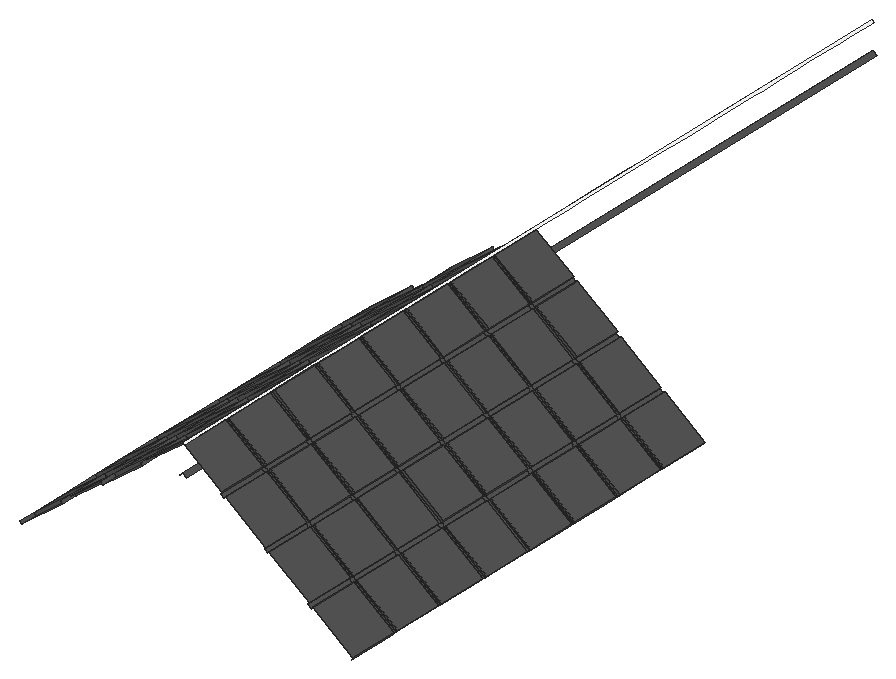
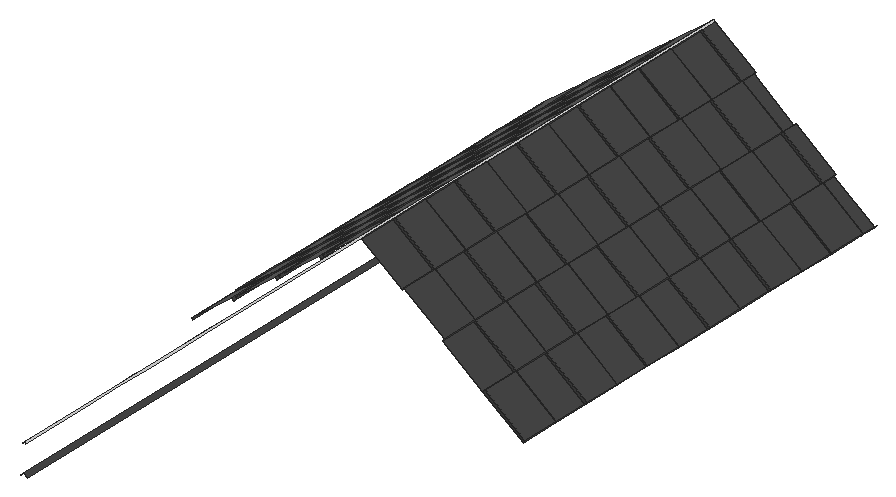
# SketchUp Ruby script. Lengths in inches.
U = 1.inch
M = Sketchup.active_model
def pt(a) = Geom::Point3d.new(a.map { |v| v * U })
def face(e, loops, mat)
  f = e.add_face(loops[0].map { |a| pt(a) })
  loops[1..].each { |l| e.add_face(l.map { |a| pt(a) }).erase! }
  f.material = f.back_material = mat if mat
  f
end
# faces: each face lists its corners as indices into pts; further lists are holes
def faces(e, pts, list, mat = nil) = list.each { |f| face(e, (f[0].is_a?(Array) ? f : [f]).map { |l| l.map { |i| pts[i] } }, mat) }
# xy, xz, yz: faces in a plane at the given z, y or x. An outline is a flat list of corners, or four numbers for a rectangle; further outlines are holes
def ring(l) = l.size == 4 ? [[l[0], l[1]], [l[2], l[1]], [l[2], l[3]], [l[0], l[3]]] : l.each_slice(2).to_a
def flat(e, list, mat, &to3) = list.each { |f| face(e, (f[0].is_a?(Array) ? f : [f]).map { |l| ring(l).map { |u, v| to3.(u, v) } }, mat) }
def xy(e, z, list, mat = nil) = flat(e, list, mat) { |x, y| [x, y, z] }
def xz(e, y, list, mat = nil) = flat(e, list, mat) { |x, z| [x, y, z] }
def yz(e, x, list, mat = nil) = flat(e, list, mat) { |y, z| [x, y, z] }
def lines(e, pts, list) = list.each { |a, b| e.add_line(pt(pts[a]), pt(pts[b])) }
# prism: a flat outline (further loops are holes) pulled along v
def prism(e, loops, v, mat = nil)
  f = face(e, loops, mat); d = Geom::Vector3d.new(v.map { |x| x * U })
  f.pushpull(f.normal.samedirection?(d) ? d.length : -d.length)
end
def box(e, o, s, mat = nil) = prism(e, [[o, [o[0] + s[0], o[1], o[2]], [o[0] + s[0], o[1] + s[1], o[2]], [o[0], o[1] + s[1], o[2]]]], [0, 0, s[2]], mat)
def at(x, y, z, deg = 0) = Geom::Transformation.translation(pt([x, y, z])) * Geom::Transformation.rotation(ORIGIN, Z_AXIS, deg.degrees)
def axes(o, x, y, z) = Geom::Transformation.new([*x, 0, *y, 0, *z, 0, *pt(o).to_a, 1])
def part(name) = M.definitions.add(name)
# library, detail: a bought-in or finely detailed component or shape, given as its bounding box
def library(name, o, s) = part(name).tap { |d| box(d.entities, o, s) }
def detail(e, o, s) = box(e.add_group.entities, o, s)
def put(e, d, t, mat = nil) = e.add_instance(d, t).tap { |i| i.material = mat if mat }
def group(e, t, mat = nil) = e.add_group.tap { |g| g.transformation = t; g.material = mat if mat }.entities
root = M.entities
M.materials.add("[Color M00]").color = [255, 255, 255]
M.materials.add("[Color M06]").color = [86, 86, 86]
xz(root,145.1875,[[301.73,378.96,320.63,393.75,320.14,394.38,319.83,394.78,300.93,379.98,301.24,379.59],[320.63,393.75,320.14,394.38,319.83,394.78,338.73,409.57,339.53,408.54],[339.53,408.54,358.43,423.34,357.63,424.36,338.73,409.57],[358.43,423.34,357.63,424.36,376.53,439.15,377.33,438.125]],"[Color M06]")
xz(root,161.375,[[456.38,376.26,437.48,391.05,438.1,391.84,457,377.05],[435.9,392.29,417,407.08,417.62,407.87,436.52,393.07],[415.43,408.3125,396.53,423.1,397.15,423.89,416.05,409.1],[394.95,424.33,377.33,438.125,377.95,438.91,395.57,425.12]],"[Color M06]")
xz(root,163.1875,[[301.73,378.96,301.24,379.59,300.93,379.98,319.83,394.78,320.14,394.38,320.63,393.75],[320.63,393.75,339.53,408.54,338.73,409.57,319.83,394.78,320.14,394.38],[339.53,408.54,338.73,409.57,357.63,424.36,358.43,423.34],[358.43,423.34,377.33,438.125,376.53,439.15,357.63,424.36]],"[Color M06]")
xz(root,163.375,[[456.38,376.26,457,377.05,438.1,391.84,437.48,391.05],[435.9,392.29,436.52,393.07,417.62,407.87,417,407.08],[415.43,408.3125,416.05,409.1,397.15,423.89,396.53,423.1],[394.95,424.33,395.57,425.12,377.95,438.91,377.33,438.125]],"[Color M06]")
xz(root,181.1875,[[301.73,378.96,320.63,393.75,320.14,394.38,319.83,394.78,300.93,379.98,301.24,379.59],[320.63,393.75,320.14,394.38,319.83,394.78,338.73,409.57,339.04,409.17,339.53,408.54],[339.53,408.54,358.43,423.34,357.9375,423.97,357.63,424.36,338.73,409.57,339.04,409.17],[358.43,423.34,357.9375,423.97,357.63,424.36,376.53,439.15,377.33,438.125]],"[Color M06]")
xz(root,187.375,[[456.38,376.26,437.48,391.05,438.1,391.84,457,377.05],[435.9,392.29,417,407.08,417.62,407.87,436.52,393.07],[415.43,408.3125,396.53,423.1,397.15,423.89,416.05,409.1],[394.95,424.33,377.33,438.125,377.95,438.91,395.57,425.12]],"[Color M06]")
xz(root,189.375,[[456.38,376.26,457,377.05,438.1,391.84,437.48,391.05],[435.9,392.29,436.52,393.07,417.62,407.87,417,407.08],[415.43,408.3125,416.05,409.1,397.15,423.89,396.53,423.1],[394.95,424.33,395.57,425.12,377.95,438.91,377.33,438.125]],"[Color M06]")
xz(root,199.1875,[[301.73,378.96,301.24,379.59,300.93,379.98,319.83,394.78,320.14,394.38,320.63,393.75],[320.63,393.75,339.53,408.54,339.04,409.17,338.73,409.57,319.83,394.78,320.14,394.38],[339.53,408.54,339.04,409.17,338.73,409.57,357.63,424.36,358.43,423.34],[358.43,423.34,377.33,438.125,376.53,439.15,357.63,424.36]],"[Color M06]")
xz(root,213.375,[[456.38,376.26,437.48,391.05,438.1,391.84,457,377.05],[435.9,392.29,417,407.08,417.62,407.87,436.52,393.07],[415.43,408.3125,396.53,423.1,397.15,423.89,416.05,409.1],[394.95,424.33,377.33,438.125,377.95,438.91,395.57,425.12]],"[Color M06]")
xz(root,215.375,[[456.38,376.26,457,377.05,438.1,391.84,437.48,391.05],[435.9,392.29,436.52,393.07,417.62,407.87,417,407.08],[415.43,408.3125,416.05,409.1,397.15,423.89,396.53,423.1],[394.95,424.33,395.57,425.12,377.95,438.91,377.33,438.125]],"[Color M06]")
xz(root,217.1875,[[301.73,378.96,320.63,393.75,320.14,394.38,319.83,394.78,300.93,379.98,301.24,379.59],[320.63,393.75,320.14,394.38,319.83,394.78,338.73,409.57,339.04,409.17,339.53,408.54],[339.53,408.54,358.43,423.34,357.63,424.36,338.73,409.57,339.04,409.17],[358.43,423.34,357.63,424.36,376.53,439.15,377.33,438.125]],"[Color M06]")
xz(root,235.1875,[[301.73,378.96,301.24,379.59,300.93,379.98,319.83,394.78,320.14,394.38,320.63,393.75],[320.63,393.75,339.53,408.54,339.04,409.17,338.73,409.57,319.83,394.78,320.14,394.38],[339.53,408.54,339.04,409.17,338.73,409.57,357.63,424.36,357.9375,423.97,358.43,423.34],[358.43,423.34,377.33,438.125,376.53,439.15,357.63,424.36,357.9375,423.97]],"[Color M06]")
xz(root,239.375,[[456.38,376.26,437.48,391.05,438.1,391.84,457,377.05],[435.9,392.29,417,407.08,417.62,407.87,436.52,393.07],[415.43,408.3125,396.53,423.1,397.15,423.89,416.05,409.1],[394.95,424.33,377.33,438.125,377.95,438.91,395.57,425.12]],"[Color M06]")
xz(root,241.375,[[456.38,376.26,457,377.05,438.1,391.84,437.48,391.05],[435.9,392.29,436.52,393.07,417.62,407.87,417,407.08],[415.43,408.3125,416.05,409.1,397.15,423.89,396.53,423.1],[394.95,424.33,395.57,425.12,377.95,438.91,377.33,438.125]],"[Color M06]")
xz(root,253.1875,[[301.73,378.96,320.63,393.75,320.14,394.38,319.83,394.78,300.93,379.98,301.24,379.59],[320.63,393.75,320.14,394.38,319.83,394.78,338.73,409.57,339.04,409.17,339.53,408.54],[339.53,408.54,358.43,423.34,357.9375,423.97,357.63,424.36,338.73,409.57,339.04,409.17],[358.43,423.34,357.9375,423.97,357.63,424.36,376.53,439.15,377.33,438.125]],"[Color M06]")
xz(root,265.375,[[456.38,376.26,437.48,391.05,438.1,391.84,457,377.05],[435.9,392.29,417,407.08,417.62,407.87,436.52,393.07],[415.43,408.3125,396.53,423.1,397.15,423.89,416.05,409.1],[394.95,424.33,377.33,438.125,377.95,438.91,395.57,425.12]],"[Color M06]")
xz(root,267.375,[[456.38,376.26,457,377.05,438.1,391.84,437.48,391.05],[435.9,392.29,436.52,393.07,417.62,407.87,417,407.08],[415.43,408.3125,416.05,409.1,397.15,423.89,396.53,423.1],[394.95,424.33,395.57,425.12,377.95,438.91,377.33,438.125]],"[Color M06]")
xz(root,271.1875,[[301.73,378.96,301.24,379.59,300.93,379.98,319.83,394.78,320.14,394.38,320.63,393.75],[320.63,393.75,339.53,408.54,339.04,409.17,338.73,409.57,319.83,394.78,320.14,394.38],[339.53,408.54,339.04,409.17,338.73,409.57,357.63,424.36,357.9375,423.97,358.43,423.34],[358.43,423.34,377.33,438.125,376.53,439.15,357.63,424.36,357.9375,423.97]],"[Color M06]")
xz(root,289.1875,[[301.73,378.96,320.63,393.75,320.14,394.38,319.83,394.78,300.93,379.98,301.24,379.59],[320.63,393.75,320.14,394.38,319.83,394.78,338.73,409.57,339.04,409.17,339.53,408.54],[339.53,408.54,358.43,423.34,357.9375,423.97,357.63,424.36,338.73,409.57,339.04,409.17],[358.43,423.34,357.9375,423.97,357.63,424.36,376.53,439.15,377.33,438.125]],"[Color M06]")
xz(root,291.375,[[456.38,376.26,437.48,391.05,438.1,391.84,457,377.05],[435.9,392.29,417,407.08,417.62,407.87,436.52,393.07],[415.43,408.3125,396.53,423.1,397.15,423.89,416.05,409.1],[394.95,424.33,377.33,438.125,377.95,438.91,395.57,425.12]],"[Color M06]")
xz(root,293.375,[[456.38,376.26,457,377.05,438.1,391.84,437.48,391.05],[435.9,392.29,436.52,393.07,417.62,407.87,417,407.08],[415.43,408.3125,416.05,409.1,397.15,423.89,396.53,423.1],[394.95,424.33,395.57,425.12,377.95,438.91,377.33,438.125]],"[Color M06]")
xz(root,307.1875,[[301.73,378.96,301.24,379.59,300.93,379.98,319.83,394.78,320.14,394.38,320.63,393.75],[320.63,393.75,339.53,408.54,339.04,409.17,338.73,409.57,319.83,394.78,320.14,394.38],[339.53,408.54,339.04,409.17,338.73,409.57,357.63,424.36,357.9375,423.97,358.43,423.34],[358.43,423.34,377.33,438.125,376.53,439.15,357.63,424.36,357.9375,423.97]],"[Color M06]")
xz(root,317.375,[[456.38,376.26,437.48,391.05,438.1,391.84,457,377.05],[435.9,392.29,417,407.08,417.62,407.87,436.52,393.07],[415.43,408.3125,396.53,423.1,397.15,423.89,416.05,409.1],[394.95,424.33,377.33,438.125,377.95,438.91,395.57,425.12]],"[Color M06]")
xz(root,319.375,[[456.38,376.26,457,377.05,438.1,391.84,437.48,391.05],[435.9,392.29,436.52,393.07,417.62,407.87,417,407.08],[415.43,408.3125,416.05,409.1,397.15,423.89,396.53,423.1],[394.95,424.33,395.57,425.12,377.95,438.91,377.33,438.125]],"[Color M06]")
xz(root,325.1875,[[301.73,378.96,320.63,393.75,319.83,394.78,300.93,379.98],[320.63,393.75,319.83,394.78,338.73,409.57,339.04,409.17,339.53,408.54],[339.53,408.54,358.43,423.34,357.9375,423.97,357.63,424.36,338.73,409.57,339.04,409.17],[358.43,423.34,357.9375,423.97,357.63,424.36,376.53,439.15,377.33,438.125]],"[Color M06]")
xz(root,343.1875,[[301.73,378.96,300.93,379.98,319.83,394.78,320.63,393.75]],"[Color M06]")
p = [[456.38,137.375,376.26],[456.38,161.375,376.26],[457,161.375,377.05],[457,137.375,377.05],[456.38,163.375,376.26],[437.48,163.375,391.05],
  [437.48,161.375,391.05],[456.38,187.375,376.26],[457,187.375,377.05],[457,163.375,377.05],[456.38,189.375,376.26],[437.48,189.375,391.05],
  [437.48,187.375,391.05],[456.38,213.375,376.26],[457,213.375,377.05],[457,189.375,377.05],[456.38,215.375,376.26],[437.48,215.375,391.05],
  [437.48,213.375,391.05],[456.38,239.375,376.26],[457,239.375,377.05],[457,215.375,377.05],[456.38,241.375,376.26],[437.48,241.375,391.05],
  [437.48,239.375,391.05],[456.38,265.375,376.26],[457,265.375,377.05],[457,241.375,377.05],[456.38,267.375,376.26],[437.48,267.375,391.05],
  [437.48,265.375,391.05],[456.38,291.375,376.26],[457,291.375,377.05],[457,267.375,377.05],[456.38,293.375,376.26],[437.48,293.375,391.05],
  [437.48,291.375,391.05],[456.38,317.375,376.26],[457,317.375,377.05],[457,293.375,377.05],[456.38,319.375,376.26],[437.48,319.375,391.05],
  [437.48,317.375,391.05],[456.38,343.375,376.26],[457,343.375,377.05],[457,319.375,377.05],[438.1,161.375,391.84],[438.1,137.375,391.84],
  [438.1,187.375,391.84],[438.1,163.375,391.84],[438.1,213.375,391.84],[438.1,189.375,391.84],[438.1,239.375,391.84],[438.1,215.375,391.84],
  [438.1,265.375,391.84],[438.1,241.375,391.84],[438.1,291.375,391.84],[438.1,267.375,391.84],[438.1,317.375,391.84],[438.1,293.375,391.84],
  [438.1,343.375,391.84],[438.1,319.375,391.84],[301.73,137.375,378.96],[301.73,145.1875,378.96],[301.24,145.1875,379.59],[300.93,145.1875,379.98],
  [300.93,137.375,379.98],[320.63,145.1875,393.75],[320.63,137.375,393.75],[301.73,163.1875,378.96],[300.93,163.1875,379.98],[301.24,163.1875,379.59],
  [301.73,181.1875,378.96],[301.24,181.1875,379.59],[300.93,181.1875,379.98],[320.63,181.1875,393.75],[320.63,163.1875,393.75],[301.73,199.1875,378.96],
  [300.93,199.1875,379.98],[301.24,199.1875,379.59],[301.73,217.1875,378.96],[301.24,217.1875,379.59],[300.93,217.1875,379.98],[320.63,217.1875,393.75],
  [320.63,199.1875,393.75],[301.73,235.1875,378.96],[300.93,235.1875,379.98],[301.24,235.1875,379.59],[301.73,253.1875,378.96],[301.24,253.1875,379.59],
  [300.93,253.1875,379.98],[320.63,253.1875,393.75],[320.63,235.1875,393.75],[301.73,271.1875,378.96],[300.93,271.1875,379.98],[301.24,271.1875,379.59],
  [301.73,289.1875,378.96],[301.24,289.1875,379.59],[300.93,289.1875,379.98],[320.63,289.1875,393.75],[320.63,271.1875,393.75],[301.73,307.1875,378.96],
  [300.93,307.1875,379.98],[301.24,307.1875,379.59],[301.73,325.1875,378.96],[300.93,325.1875,379.98],[320.63,325.1875,393.75],[320.63,307.1875,393.75],
  [301.73,343.1875,378.96],[300.93,343.1875,379.98],[319.83,163.1875,394.78],[319.83,145.1875,394.78],[319.83,199.1875,394.78],[319.83,181.1875,394.78],
  [319.83,235.1875,394.78],[319.83,217.1875,394.78],[319.83,271.1875,394.78],[319.83,253.1875,394.78],[319.83,307.1875,394.78],[319.83,289.1875,394.78],
  [319.83,343.1875,394.78],[319.83,325.1875,394.78],[435.9,161.375,392.29],[435.9,137.375,392.29],[437.48,137.375,391.05],[435.9,163.375,392.29],
  [435.9,187.375,392.29],[435.9,189.375,392.29],[435.9,213.375,392.29],[435.9,215.375,392.29],[435.9,239.375,392.29],[435.9,241.375,392.29],
  [435.9,265.375,392.29],[435.9,267.375,392.29],[435.9,291.375,392.29],[435.9,293.375,392.29],[435.9,317.375,392.29],[435.9,319.375,392.29],
  [437.48,343.375,391.05],[435.9,343.375,392.29],[436.52,161.375,393.07],[436.52,137.375,393.07],[417,163.375,407.08],[417,161.375,407.08],
  [436.52,187.375,393.07],[436.52,163.375,393.07],[417,189.375,407.08],[417,187.375,407.08],[436.52,213.375,393.07],[436.52,189.375,393.07],
  [417,215.375,407.08],[417,213.375,407.08],[436.52,239.375,393.07],[436.52,215.375,393.07],[417,241.375,407.08],[417,239.375,407.08],
  [436.52,265.375,393.07],[436.52,241.375,393.07],[417,267.375,407.08],[417,265.375,407.08],[436.52,291.375,393.07],[436.52,267.375,393.07],
  [417,293.375,407.08],[417,291.375,407.08],[436.52,317.375,393.07],[436.52,293.375,393.07],[417,319.375,407.08],[417,317.375,407.08],
  [436.52,343.375,393.07],[436.52,319.375,393.07],[417.62,161.375,407.87],[417.62,137.375,407.87],[417.62,187.375,407.87],[417.62,163.375,407.87],
  [417.62,213.375,407.87],[417.62,189.375,407.87],[417.62,239.375,407.87],[417.62,215.375,407.87],[417.62,265.375,407.87],[417.62,241.375,407.87],
  [417.62,291.375,407.87],[417.62,267.375,407.87],[417.62,317.375,407.87],[417.62,293.375,407.87],[417.62,343.375,407.87],[417.62,319.375,407.87],
  [319.83,137.375,394.78],[320.14,145.1875,394.38],[320.14,163.1875,394.38],[339.53,163.1875,408.54],[339.53,145.1875,408.54],[320.14,181.1875,394.38],
  [320.14,199.1875,394.38],[339.53,199.1875,408.54],[339.53,181.1875,408.54],[320.14,217.1875,394.38],[320.14,235.1875,394.38],[339.53,235.1875,408.54],
  [339.53,217.1875,408.54],[320.14,253.1875,394.38],[320.14,271.1875,394.38],[339.53,271.1875,408.54],[339.53,253.1875,408.54],[320.14,289.1875,394.38],
  [320.14,307.1875,394.38],[339.53,307.1875,408.54],[339.53,289.1875,408.54],[320.63,343.1875,393.75],[339.53,343.1875,408.54],[339.53,325.1875,408.54],
  [338.73,145.1875,409.57],[338.73,137.375,409.57],[338.73,181.1875,409.57],[338.73,163.1875,409.57],[338.73,217.1875,409.57],[338.73,199.1875,409.57],
  [338.73,253.1875,409.57],[338.73,235.1875,409.57],[338.73,289.1875,409.57],[338.73,271.1875,409.57],[338.73,325.1875,409.57],[338.73,307.1875,409.57],
  [415.43,161.375,408.3125],[415.43,137.375,408.3125],[417,137.375,407.08],[415.43,163.375,408.3125],[415.43,187.375,408.3125],[415.43,189.375,408.3125],
  [415.43,213.375,408.3125],[415.43,215.375,408.3125],[415.43,239.375,408.3125],[415.43,241.375,408.3125],[415.43,265.375,408.3125],[415.43,267.375,408.3125],
  [415.43,291.375,408.3125],[415.43,293.375,408.3125],[415.43,317.375,408.3125],[415.43,319.375,408.3125],[417,343.375,407.08],[415.43,343.375,408.3125],
  [416.05,161.375,409.1],[416.05,137.375,409.1],[396.53,163.375,423.1],[396.53,161.375,423.1],[416.05,187.375,409.1],[416.05,163.375,409.1],
  [396.53,189.375,423.1],[396.53,187.375,423.1],[416.05,213.375,409.1],[416.05,189.375,409.1],[396.53,215.375,423.1],[396.53,213.375,423.1],
  [416.05,239.375,409.1],[416.05,215.375,409.1],[396.53,241.375,423.1],[396.53,239.375,423.1],[416.05,265.375,409.1],[416.05,241.375,409.1],
  [396.53,267.375,423.1],[396.53,265.375,423.1],[416.05,291.375,409.1],[416.05,267.375,409.1],[396.53,293.375,423.1],[396.53,291.375,423.1],
  [416.05,317.375,409.1],[416.05,293.375,409.1],[396.53,319.375,423.1],[396.53,317.375,423.1],[416.05,343.375,409.1],[416.05,319.375,409.1],
  [339.53,137.375,408.54],[358.43,145.1875,423.34],[358.43,137.375,423.34],[339.04,181.1875,409.17],[358.43,181.1875,423.34],[358.43,163.1875,423.34],
  [339.04,199.1875,409.17],[339.04,217.1875,409.17],[358.43,217.1875,423.34],[358.43,199.1875,423.34],[339.04,235.1875,409.17],[339.04,253.1875,409.17],
  [358.43,253.1875,423.34],[358.43,235.1875,423.34],[339.04,271.1875,409.17],[339.04,289.1875,409.17],[358.43,289.1875,423.34],[358.43,271.1875,423.34],
  [339.04,307.1875,409.17],[339.04,325.1875,409.17],[358.43,325.1875,423.34],[358.43,307.1875,423.34],[338.73,343.1875,409.57],[339.04,343.1875,409.17],
  [397.15,161.375,423.89],[397.15,137.375,423.89],[397.15,187.375,423.89],[397.15,163.375,423.89],[397.15,213.375,423.89],[397.15,189.375,423.89],
  [397.15,239.375,423.89],[397.15,215.375,423.89],[397.15,265.375,423.89],[397.15,241.375,423.89],[397.15,291.375,423.89],[397.15,267.375,423.89],
  [397.15,317.375,423.89],[397.15,293.375,423.89],[397.15,343.375,423.89],[397.15,319.375,423.89],[357.63,163.1875,424.36],[357.63,145.1875,424.36],
  [357.63,199.1875,424.36],[357.63,181.1875,424.36],[357.63,235.1875,424.36],[357.63,217.1875,424.36],[357.63,271.1875,424.36],[357.63,253.1875,424.36],
  [357.63,307.1875,424.36],[357.63,289.1875,424.36],[357.63,343.1875,424.36],[357.63,325.1875,424.36],[394.95,161.375,424.33],[394.95,137.375,424.33],
  [396.53,137.375,423.1],[394.95,163.375,424.33],[394.95,187.375,424.33],[394.95,189.375,424.33],[394.95,213.375,424.33],[394.95,215.375,424.33],
  [394.95,239.375,424.33],[394.95,241.375,424.33],[394.95,265.375,424.33],[394.95,267.375,424.33],[394.95,291.375,424.33],[394.95,293.375,424.33],
  [394.95,317.375,424.33],[394.95,319.375,424.33],[396.53,343.375,423.1],[394.95,343.375,424.33],[357.63,137.375,424.36],[377.33,163.1875,438.125],
  [377.33,145.1875,438.125],[377.33,161.375,438.125],[357.9375,181.1875,423.97],[377.33,163.375,438.125],[377.33,181.1875,438.125],[377.33,199.1875,438.125],
  [377.33,187.375,438.125],[377.33,189.375,438.125],[357.9375,235.1875,423.97],[377.33,235.1875,438.125],[377.33,217.1875,438.125],[357.9375,253.1875,423.97],
  [357.9375,271.1875,423.97],[377.33,271.1875,438.125],[377.33,253.1875,438.125],[377.33,265.375,438.125],[377.33,267.375,438.125],[357.9375,289.1875,423.97],
  [357.9375,307.1875,423.97],[377.33,307.1875,438.125],[377.33,289.1875,438.125],[377.33,291.375,438.125],[377.33,293.375,438.125],[357.9375,325.1875,423.97],
  [358.43,343.1875,423.34],[357.9375,343.1875,423.97],[377.33,343.1875,438.125],[377.33,325.1875,438.125],[395.57,161.375,425.12],[395.57,137.375,425.12],
  [395.57,187.375,425.12],[395.57,163.375,425.12],[395.57,213.375,425.12],[395.57,189.375,425.12],[377.33,213.375,438.125],[377.33,215.375,438.125],
  [395.57,239.375,425.12],[395.57,215.375,425.12],[377.33,239.375,438.125],[377.33,241.375,438.125],[395.57,265.375,425.12],[395.57,241.375,425.12],
  [395.57,291.375,425.12],[395.57,267.375,425.12],[395.57,317.375,425.12],[395.57,293.375,425.12],[377.33,317.375,438.125],[377.33,319.375,438.125],
  [395.57,343.375,425.12],[395.57,319.375,425.12],[376.53,145.1875,439.15],[376.53,137.375,439.15],[376.53,181.1875,439.15],[376.53,163.1875,439.15],
  [376.53,217.1875,439.15],[376.53,199.1875,439.15],[376.53,253.1875,439.15],[376.53,235.1875,439.15],[376.53,289.1875,439.15],[376.53,271.1875,439.15],
  [376.53,325.1875,439.15],[376.53,307.1875,439.15],[377.95,137.375,438.91],[377.95,161.375,438.91],[377.95,145.1875,438.91],[377.95,163.375,438.91],
  [377.95,187.375,438.91],[377.95,181.1875,438.91],[377.95,189.375,438.91],[377.95,213.375,438.91],[377.95,199.1875,438.91],[377.95,215.375,438.91],
  [377.95,239.375,438.91],[377.95,235.1875,438.91],[377.95,217.1875,438.91],[377.95,241.375,438.91],[377.95,265.375,438.91],[377.95,253.1875,438.91],
  [377.95,267.375,438.91],[377.95,291.375,438.91],[377.95,289.1875,438.91],[377.95,271.1875,438.91],[377.95,293.375,438.91],[377.95,317.375,438.91],
  [377.95,307.1875,438.91],[377.95,319.375,438.91],[377.95,343.375,438.91],[377.95,343.1875,438.91],[377.95,325.1875,438.91],[377.33,137.375,426.7],
  [375.48,137.375,425.25],[375.48,541.1875,425.25],[377.33,541.1875,426.7],[379.18,137.375,425.25],[379.18,541.1875,425.25],[376.68,317.375,438.63],
  [376.68,319.375,438.63],[376.53,343.1875,439.15],[377.09,137.375,439.59],[377.09,541.1875,439.59],[377.95,541.1875,438.91],[377.95,525.375,438.91],
  [377.95,523.1875,438.91],[377.95,505.1875,438.91],[377.95,501.375,438.91],[377.95,499.375,438.91],[377.95,487.1875,438.91],[377.95,475.375,438.91],
  [377.95,473.375,438.91],[377.95,469.1875,438.91],[377.95,451.1875,438.91],[377.95,449.375,438.91],[377.95,447.375,438.91],[377.95,433.1875,438.91],
  [377.95,423.375,438.91],[377.95,421.375,438.91],[377.95,415.1875,438.91],[377.95,397.375,438.91],[377.95,395.375,438.91],[377.95,379.1875,438.91],
  [377.95,371.375,438.91],[377.95,369.375,438.91],[377.95,361.1875,438.91],[377.95,345.375,438.91],[376.53,361.1875,439.15],[376.53,379.1875,439.15],
  [376.53,397.1875,439.15],[376.53,415.1875,439.15],[376.53,433.1875,439.15],[376.53,451.1875,439.15],[376.53,469.1875,439.15],[376.53,487.1875,439.15],
  [376.53,505.1875,439.15],[376.53,523.1875,439.15],[376.53,541.1875,439.15],[377.33,137.375,438.125]]
faces(root,p,[[0,1,2,3],[4,5,6,1],[4,7,8,9],[10,11,12,7],[10,13,14,15],[16,17,18,13],[16,19,20,21],[22,23,24,19],
  [22,25,26,27],[28,29,30,25],[28,31,32,33],[34,35,36,31],[34,37,38,39],[40,41,42,37],[40,43,44,45],[2,46,47,3],
  [8,48,49,9],[14,50,51,15],[20,52,53,21],[26,54,55,27],[32,56,57,33],[38,58,59,39],[44,60,61,45],[62,63,64,65,66],
  [67,63,62,68],[69,63,64,65,70,71],[69,72,73,74,70,71],[75,72,69,76],[77,72,73,74,78,79],[77,80,81,82,78,79],[83,80,77,84],[85,80,81,82,86,87],
  [85,88,89,90,86,87],[91,88,85,92],[93,88,89,90,94,95],[93,96,97,98,94,95],[99,96,93,100],[101,96,97,98,102,103],[101,104,105,102,103],[106,104,101,107],
  [108,104,105,109],[110,70,65,111],[112,78,74,113],[114,86,82,115],[116,94,90,117],[118,102,98,119],[120,109,105,121],[6,122,123,124],
  [6,124,47,46],[122,6,5,125],[12,126,125,5],[12,5,49,48],[11,127,126,12],[127,11,18,128],[18,11,51,50],[17,129,128,18],
  [129,17,24,130],[24,17,53,52],[130,24,23,131],[30,132,131,23],[30,23,55,54],[132,30,29,133],[133,29,36,134],[36,29,57,56],
  [35,135,134,36],[42,136,135,35],[42,35,59,58],[136,42,41,137],[137,41,138,139],[138,41,61,60],[123,122,140,141],[125,142,143,122],
  [125,126,144,145],[127,146,147,126],[127,128,148,149],[129,150,151,128],[129,130,152,153],[131,154,155,130],[131,132,156,157],[133,158,159,132],
  [133,134,160,161],[135,162,163,134],[135,136,164,165],[137,166,167,136],[137,139,168,169],[140,170,171,141],[144,172,173,145],[148,174,175,149],
  [152,176,177,153],[156,178,179,157],[160,180,181,161],[164,182,183,165],[168,184,185,169],[67,68,186,111,187],[67,76,188,110,111,187],[189,76,67,190],
  [75,76,188,110,113,191],[75,84,192,112,113,191],[193,84,75,194],[83,84,192,112,115,195],[83,92,196,114,115,195],[197,92,83,198],[91,92,196,114,117,199],[91,100,200,116,117,199],
  [201,100,91,202],[99,100,200,116,119,203],[99,107,204,118,119,203],[205,107,99,206],[106,107,204,118,121],[106,207,120,121],[208,207,106,209],[210,111,186,211],
  [212,113,110,213],[214,115,112,215],[216,117,114,217],[218,119,116,219],[220,121,118,221],[143,222,223,224],[143,224,171,170],[142,225,222,143],
  [225,142,147,226],[147,142,173,172],[226,147,146,227],[227,146,151,228],[151,146,175,174],[150,229,228,151],[155,230,229,150],[155,150,177,176],
  [230,155,154,231],[159,232,231,154],[159,154,179,178],[232,159,158,233],[233,158,163,234],[163,158,181,180],[234,163,162,235],[167,236,235,162],
  [167,162,183,182],[166,237,236,167],[237,166,238,239],[238,166,185,184],[223,222,240,241],[225,242,243,222],[225,226,244,245],[227,246,247,226],
  [227,228,248,249],[229,250,251,228],[229,230,252,253],[231,254,255,230],[231,232,256,257],[233,258,259,232],[233,234,260,261],[235,262,263,234],
  [235,236,264,265],[237,266,267,236],[237,239,268,269],[270,190,210,211],[271,190,270,272],[189,190,210,213],[189,194,273,212,213],[274,194,189,275],
  [193,194,273,212,215,276],[193,198,277,214,215,276],[278,198,193,279],[197,198,277,214,217,280],[197,202,281,216,217,280],[282,202,197,283],[201,202,281,216,219,284],[201,206,285,218,219,284],
  [286,206,201,287],[205,206,285,218,221,288],[205,209,289,220,221,288],[290,209,205,291],[208,209,289,220,292,293],[240,294,295,241],[244,296,297,245],[248,298,299,249],
  [252,300,301,253],[256,302,303,257],[260,304,305,261],[264,306,307,265],[268,308,309,269],[310,213,210,311],[312,215,212,313],[314,217,214,315],
  [316,219,216,317],[318,221,218,319],[320,292,220,321],[243,322,323,324],[243,324,295,294],[242,325,322,243],[247,326,325,242],[247,242,297,296],
  [246,327,326,247],[251,328,327,246],[251,246,299,298],[250,329,328,251],[255,330,329,250],[255,250,301,300],[330,255,254,331],[259,332,331,254],
  [259,254,303,302],[332,259,258,333],[333,258,263,334],[263,258,305,304],[334,263,262,335],[267,336,335,262],[267,262,307,306],[266,337,336,267],
  [338,339,337,266],[338,266,309,308],[271,272,340,311],[271,275,310,311],[341,275,271,342,343],[274,275,310,313,344],[341,345,346,274,275],[274,279,312,313,344],
  [347,279,274,346,348,349],[278,279,312,315],[278,283,350,314,315],[351,283,278,352],[282,283,350,314,317,353],[282,287,354,316,317,353],[355,287,282,356,357,358],[286,287,354,316,319,359],
  [286,291,360,318,319,359],[361,291,286,362,363,364],[290,291,360,318,321,365],[290,366,367,320,321,365],[368,366,290,369],[323,322,370,371],[343,322,325,345,341],[325,326,372,373],
  [348,326,327,349],[327,328,374,375],[376,328,329,377],[329,330,378,379],[380,330,331,381],[331,332,382,383],[357,332,333,358],[333,334,384,385],
  [363,334,335,364],[335,336,386,387],[388,336,337,389],[337,339,390,391],[392,311,340,393],[394,313,310,395],[396,315,312,397],[398,317,314,399],
  [400,319,316,401],[402,321,318,403],[404,371,370,405,406],[407,373,372,408,409],[410,375,374,411,412],[413,379,378,414,415,416],[417,383,382,418,419],[420,385,384,421,422,423],
  [424,387,386,425,426],[427,391,390,428,429,430],[431,432,433,434],[435,431,434,436],[343,341,395,392,342],[343,342,406,405],[405,407,345,341,343],[341,345,346,394,395],
  [346,345,407,409],[397,394,346,348,349,347],[348,346,409,408],[349,348,408,410],[347,349,410,412],[347,376,377,352,396,397],[376,347,412,411],[377,376,411,413],
  [352,377,413,416],[399,396,352,351],[351,352,416,415],[351,380,381,356,398,399],[380,351,415,414],[381,380,414,417],[356,381,417,419],[401,398,356,357,358,355],
  [357,356,419,418],[358,357,418,420],[355,358,420,423],[355,362,400,401],[362,355,423,422],[403,400,362,363,364,361],[363,362,422,421],[364,363,421,424],
  [361,364,424,426],[361,388,389,369,402,403],[388,361,426,425],[437,388,389,438],[389,388,425,427],[369,389,427,430],[439,402,369,368],[368,369,430,429]],"[Color M06]")
faces(root,p,[[404,440,441,442,443,444,445,446,447,448,449,450,451,452,453,454,455,456,457,458,459,460,461,462,463,464,465,428,429,430,427,425,426,424,421,422,423,420,418,419,417,414,415,416,413,411,412,410,408,409,407,405,406],[440,393,392,395,394,397,396,399,398,401,400,403,402,439,466,467,468,469,470,471,472,473,474,475,476,441]],"[Color M00]")
lines(root,p,[[477,342]])
